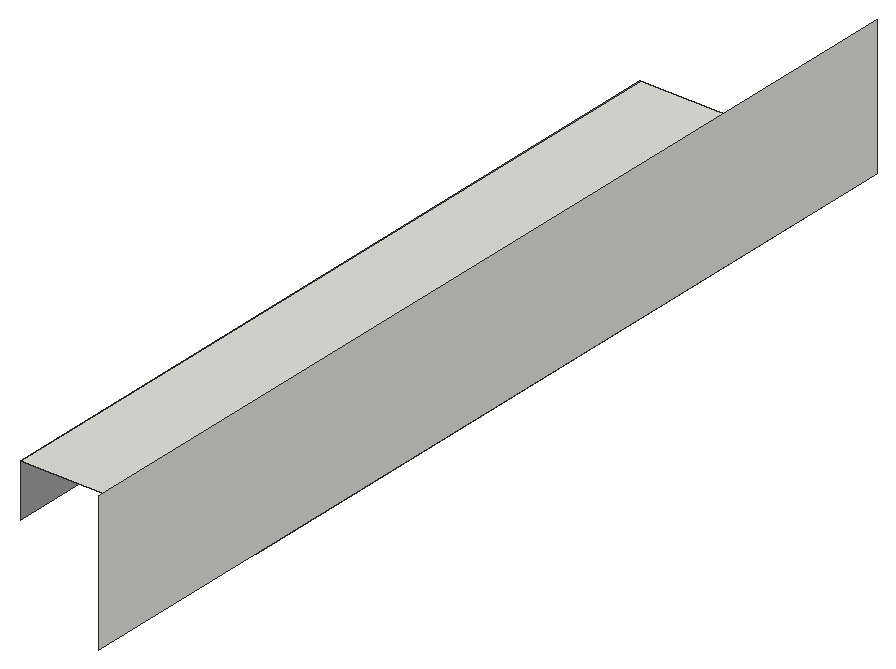
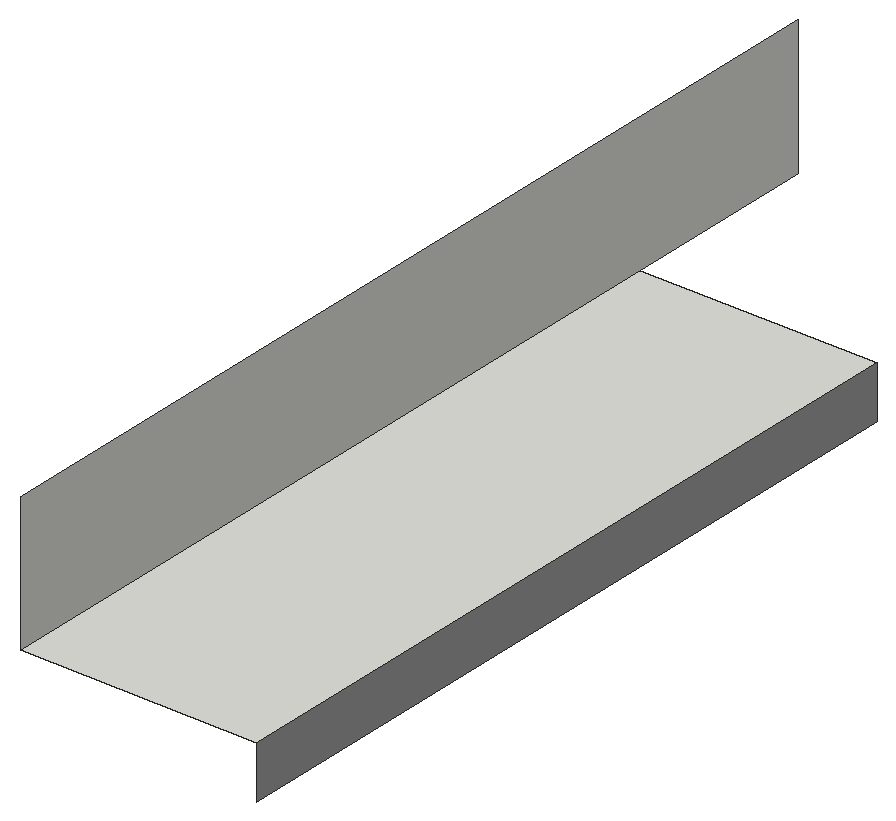
# SketchUp Ruby script. Lengths in inches.
U = 1.inch
M = Sketchup.active_model
def pt(a) = Geom::Point3d.new(a.map { |v| v * U })
def face(e, loops, mat)
  f = e.add_face(loops[0].map { |a| pt(a) })
  loops[1..].each { |l| e.add_face(l.map { |a| pt(a) }).erase! }
  f.material = f.back_material = mat if mat
  f
end
# faces: each face lists its corners as indices into pts; further lists are holes
def faces(e, pts, list, mat = nil) = list.each { |f| face(e, (f[0].is_a?(Array) ? f : [f]).map { |l| l.map { |i| pts[i] } }, mat) }
# xy, xz, yz: faces in a plane at the given z, y or x. An outline is a flat list of corners, or four numbers for a rectangle; further outlines are holes
def ring(l) = l.size == 4 ? [[l[0], l[1]], [l[2], l[1]], [l[2], l[3]], [l[0], l[3]]] : l.each_slice(2).to_a
def flat(e, list, mat, &to3) = list.each { |f| face(e, (f[0].is_a?(Array) ? f : [f]).map { |l| ring(l).map { |u, v| to3.(u, v) } }, mat) }
def xy(e, z, list, mat = nil) = flat(e, list, mat) { |x, y| [x, y, z] }
def xz(e, y, list, mat = nil) = flat(e, list, mat) { |x, z| [x, y, z] }
def yz(e, x, list, mat = nil) = flat(e, list, mat) { |y, z| [x, y, z] }
def lines(e, pts, list) = list.each { |a, b| e.add_line(pt(pts[a]), pt(pts[b])) }
# prism: a flat outline (further loops are holes) pulled along v
def prism(e, loops, v, mat = nil)
  f = face(e, loops, mat); d = Geom::Vector3d.new(v.map { |x| x * U })
  f.pushpull(f.normal.samedirection?(d) ? d.length : -d.length)
end
def box(e, o, s, mat = nil) = prism(e, [[o, [o[0] + s[0], o[1], o[2]], [o[0] + s[0], o[1] + s[1], o[2]], [o[0], o[1] + s[1], o[2]]]], [0, 0, s[2]], mat)
def at(x, y, z, deg = 0) = Geom::Transformation.translation(pt([x, y, z])) * Geom::Transformation.rotation(ORIGIN, Z_AXIS, deg.degrees)
def axes(o, x, y, z) = Geom::Transformation.new([*x, 0, *y, 0, *z, 0, *pt(o).to_a, 1])
def part(name) = M.definitions.add(name)
# library, detail: a bought-in or finely detailed component or shape, given as its bounding box
def library(name, o, s) = part(name).tap { |d| box(d.entities, o, s) }
def detail(e, o, s) = box(e.add_group.entities, o, s)
def put(e, d, t, mat = nil) = e.add_instance(d, t).tap { |i| i.material = mat if mat }
def group(e, t, mat = nil) = e.add_group.tap { |g| g.transformation = t; g.material = mat if mat }.entities
root = M.entities
M.materials.add("[Blinds Vertical Stripe Gray]").color = [160, 160, 160]
xy(root,58.8125,[[206.19,96.24,210.69,111]])
yz(root,206.19,[[96.24,57.8125,111,58.8125]],"[Blinds Vertical Stripe Gray]")
yz(root,210.69,[[92.49,58.8125,111,61.4375]])
